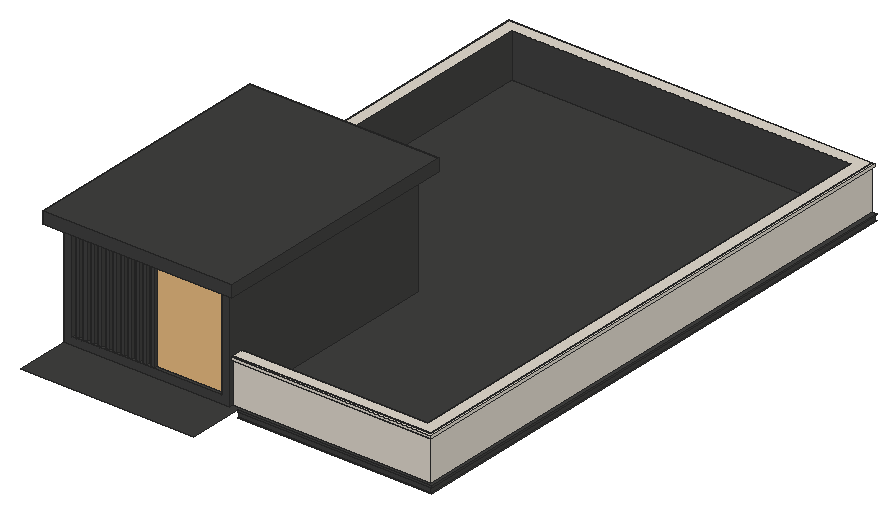
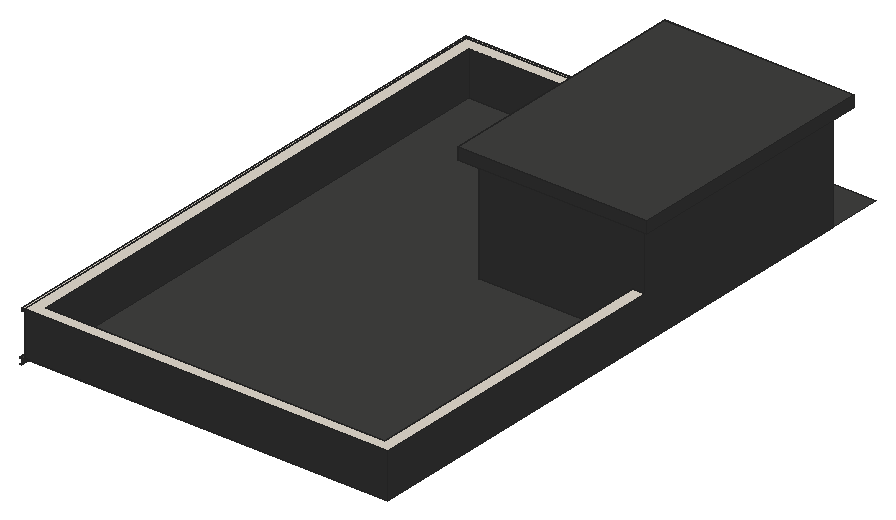
# SketchUp Ruby script. Lengths in inches.
U = 1.inch
M = Sketchup.active_model
def pt(a) = Geom::Point3d.new(a.map { |v| v * U })
def face(e, loops, mat)
  f = e.add_face(loops[0].map { |a| pt(a) })
  loops[1..].each { |l| e.add_face(l.map { |a| pt(a) }).erase! }
  f.material = f.back_material = mat if mat
  f
end
# faces: each face lists its corners as indices into pts; further lists are holes
def faces(e, pts, list, mat = nil) = list.each { |f| face(e, (f[0].is_a?(Array) ? f : [f]).map { |l| l.map { |i| pts[i] } }, mat) }
# xy, xz, yz: faces in a plane at the given z, y or x. An outline is a flat list of corners, or four numbers for a rectangle; further outlines are holes
def ring(l) = l.size == 4 ? [[l[0], l[1]], [l[2], l[1]], [l[2], l[3]], [l[0], l[3]]] : l.each_slice(2).to_a
def flat(e, list, mat, &to3) = list.each { |f| face(e, (f[0].is_a?(Array) ? f : [f]).map { |l| ring(l).map { |u, v| to3.(u, v) } }, mat) }
def xy(e, z, list, mat = nil) = flat(e, list, mat) { |x, y| [x, y, z] }
def xz(e, y, list, mat = nil) = flat(e, list, mat) { |x, z| [x, y, z] }
def yz(e, x, list, mat = nil) = flat(e, list, mat) { |y, z| [x, y, z] }
def lines(e, pts, list) = list.each { |a, b| e.add_line(pt(pts[a]), pt(pts[b])) }
# prism: a flat outline (further loops are holes) pulled along v
def prism(e, loops, v, mat = nil)
  f = face(e, loops, mat); d = Geom::Vector3d.new(v.map { |x| x * U })
  f.pushpull(f.normal.samedirection?(d) ? d.length : -d.length)
end
def box(e, o, s, mat = nil) = prism(e, [[o, [o[0] + s[0], o[1], o[2]], [o[0] + s[0], o[1] + s[1], o[2]], [o[0], o[1] + s[1], o[2]]]], [0, 0, s[2]], mat)
def at(x, y, z, deg = 0) = Geom::Transformation.translation(pt([x, y, z])) * Geom::Transformation.rotation(ORIGIN, Z_AXIS, deg.degrees)
def axes(o, x, y, z) = Geom::Transformation.new([*x, 0, *y, 0, *z, 0, *pt(o).to_a, 1])
def part(name) = M.definitions.add(name)
# library, detail: a bought-in or finely detailed component or shape, given as its bounding box
def library(name, o, s) = part(name).tap { |d| box(d.entities, o, s) }
def detail(e, o, s) = box(e.add_group.entities, o, s)
def put(e, d, t, mat = nil) = e.add_instance(d, t).tap { |i| i.material = mat if mat }
def group(e, t, mat = nil) = e.add_group.tap { |g| g.transformation = t; g.material = mat if mat }.entities
root = M.entities
M.materials.add("1448 AP 8253 RAVEN SONG").color = [64, 64, 63]
M.materials.add("Wall Light").color = [250, 218, 132]
M.materials.add("[Tile Various Tan]").color = [223, 216, 204]
c1 = part("2")
box(c1.entities,[0,0,0],[3,2,70])
c2 = library("PF4VTX2R\#1",[0,-0.39,0],[145.67,4.18,85.83])
xy(root,472,[[142.14,237,290.46,237,290.46,663,289.43,663,289.43,238,142.14,238]],"1448 AP 8253 RAVEN SONG")
xy(root,474,[[39.3,217.5,39.23,217.51,39.15,217.52,39.07,217.52,38.99,217.54,38.91,217.55,38.84,217.5625,38.76,217.58,38.68,217.6,38.61,217.62,38.53,217.64,38.39,217.7,38.3125,217.72,38.24,217.75,38.17,217.79,38.1,217.82,37.96,217.9,37.89,217.9375,37.83,217.98,37.76,218.02,37.7,218.07,37.63,218.11,37.45,218.26,37.23,218.48,37.18,218.54,37.125,218.6,37.08,218.66,37.03,218.73,36.98,218.79,36.94,218.86,36.9,218.92,36.78,219.13,36.75,219.2,36.71,219.27,36.65,219.41,36.625,219.49,36.6,219.5625,36.58,219.64,36.56,219.71,36.52,219.87,36.5,219.94,36.47,220.18,36.46,220.25,36.45,220.33,36.45,220.65,36.46,220.72,36.47,220.8,36.47,220.88,36.49,220.96,36.5,221.04,36.51,221.11,36.53,221.1875,36.55,221.27,36.57,221.34,36.59,221.42,36.62,221.49,36.65,221.5625,36.67,221.64,36.7,221.71,36.74,221.78,36.77,221.85,36.89,222.06,36.97,222.19,37.02,222.25,37.0625,222.32,37.11,222.38,37.21,222.5,37.32,222.61,37.375,222.67,37.43,222.72,37.55,222.82,37.61,222.875,37.68,222.92,37.74,222.97,37.81,223.01,37.87,223.05,38.08,223.17,38.15,223.2,38.22,223.24,38.36,223.3,38.4375,223.32,38.51,223.35,38.59,223.375,38.66,223.39,38.82,223.43,38.89,223.45,39.05,223.47,39.2,223.49,39.28,223.5,39.6,223.5,39.67,223.49,39.75,223.48,39.83,223.48,39.91,223.46,39.99,223.45,40.0625,223.4375,40.14,223.42,40.22,223.4,40.29,223.38,40.37,223.36,40.51,223.3,40.59,223.28,40.66,223.25,40.73,223.21,40.8,223.18,40.94,223.1,41.01,223.0625,41.07,223.02,41.14,222.98,41.2,222.93,41.27,222.89,41.45,222.74,41.51,222.68,41.5625,222.63,41.62,222.57,41.67,222.52,41.82,222.34,41.87,222.27,41.92,222.21,41.96,222.14,42,222.08,42.12,221.87,42.15,221.8,42.1875,221.73,42.22,221.66,42.25,221.59,42.27,221.51,42.3,221.4375,42.32,221.36,42.34,221.29,42.38,221.13,42.4,221.06,42.43,220.82,42.44,220.75,42.45,220.67,42.45,220.35,42.44,220.28,42.43,220.2,42.43,220.12,42.41,220.04,42.4,219.96,42.39,219.89,42.37,219.8125,42.35,219.73,42.33,219.66,42.31,219.58,42.28,219.51,42.25,219.4375,42.23,219.36,42.2,219.29,42.16,219.22,42.13,219.15,42.01,218.94,41.93,218.81,41.88,218.75,41.84,218.68,41.74,218.56,41.6875,218.5,41.63,218.44,41.47,218.28,41.35,218.18,41.29,218.125,41.22,218.08,41.16,218.03,41.09,217.99,41.03,217.95,40.82,217.83,40.75,217.8,40.68,217.76,40.54,217.7,40.46,217.68,40.39,217.65,40.3125,217.625,40.24,217.61,40.08,217.57,40.01,217.55,39.77,217.52,39.7,217.51,39.62,217.5],[117.99,217.5,117.92,217.51,117.84,217.52,117.76,217.52,117.68,217.54,117.6,217.55,117.53,217.5625,117.45,217.58,117.3,217.62,117.22,217.64,117.08,217.7,117,217.72,116.93,217.75,116.86,217.79,116.79,217.82,116.65,217.9,116.58,217.9375,116.52,217.98,116.45,218.02,116.39,218.07,116.32,218.11,116.14,218.26,115.92,218.48,115.77,218.66,115.72,218.73,115.67,218.79,115.63,218.86,115.59,218.92,115.47,219.13,115.4375,219.2,115.4,219.27,115.34,219.41,115.32,219.49,115.29,219.5625,115.27,219.64,115.25,219.71,115.21,219.87,115.19,219.94,115.16,220.18,115.15,220.25,115.14,220.33,115.14,220.65,115.15,220.72,115.16,220.8,115.16,220.88,115.18,220.96,115.1875,221.04,115.2,221.11,115.22,221.1875,115.24,221.27,115.26,221.34,115.28,221.42,115.31,221.49,115.34,221.5625,115.36,221.64,115.39,221.71,115.43,221.78,115.46,221.85,115.58,222.06,115.66,222.19,115.71,222.25,115.75,222.32,115.9,222.5,116.07,222.67,116.18,222.77,116.24,222.82,116.3,222.875,116.37,222.92,116.43,222.97,116.5,223.01,116.5625,223.05,116.63,223.09,116.77,223.17,116.84,223.2,116.91,223.24,117.05,223.3,117.13,223.32,117.2,223.35,117.28,223.375,117.35,223.39,117.51,223.43,117.58,223.45,117.82,223.48,117.89,223.49,117.97,223.5,118.29,223.5,118.36,223.49,118.44,223.48,118.52,223.48,118.6,223.46,118.68,223.45,118.75,223.4375,118.83,223.42,118.91,223.4,118.98,223.38,119.06,223.36,119.2,223.3,119.28,223.28,119.35,223.25,119.42,223.21,119.49,223.18,119.5625,223.14,119.63,223.1,119.7,223.0625,119.76,223.02,119.83,222.98,119.89,222.93,119.96,222.89,120.14,222.74,120.36,222.52,120.51,222.34,120.56,222.27,120.61,222.21,120.65,222.14,120.69,222.08,120.81,221.87,120.84,221.8,120.91,221.66,120.9375,221.59,120.96,221.51,120.99,221.4375,121.01,221.36,121.03,221.29,121.07,221.13,121.09,221.06,121.12,220.82,121.13,220.75,121.14,220.67,121.14,220.35,121.13,220.28,121.12,220.12,121.1,220.04,121.09,219.96,121.08,219.89,121.06,219.8125,121.04,219.73,121.02,219.66,121,219.58,120.97,219.51,120.94,219.4375,120.92,219.36,120.89,219.29,120.85,219.22,120.82,219.15,120.7,218.94,120.62,218.81,120.57,218.75,120.53,218.68,120.38,218.5,120.16,218.28,120.04,218.18,119.98,218.125,119.91,218.08,119.85,218.03,119.78,217.99,119.72,217.95,119.51,217.83,119.44,217.8,119.37,217.76,119.23,217.7,119.15,217.68,119.08,217.65,119,217.625,118.93,217.61,118.77,217.57,118.7,217.55,118.46,217.52,118.39,217.51,118.31,217.5]],"1448 AP 8253 RAVEN SONG")
xy(root,476,[[142.14,237,142.14,238,289.43,238,289.43,663,290.46,663,290.46,237]],"1448 AP 8253 RAVEN SONG")
xy(root,477,[[9.27,195,142.14,195,142.14,237,290.46,237,290.46,663,9.27,663]],"1448 AP 8253 RAVEN SONG")
xz(root,217.5,[[39.3,471,39.38,474],[39.38,471,39.46,474],[39.46,471,39.54,474],[39.54,471,39.62,474]],"1448 AP 8253 RAVEN SONG")
xz(root,217.52,[[39.07,471,39.15,474]],"1448 AP 8253 RAVEN SONG")
xz(root,223.48,[[39.75,471,39.83,474]],"1448 AP 8253 RAVEN SONG")
xz(root,223.5,[[39.28,471,39.36,474],[39.36,471,39.4375,474],[39.4375,471,39.52,474],[39.52,471,39.6,474]],"1448 AP 8253 RAVEN SONG")
xz(root,237,[[142.14,476,290.46,477]],"1448 AP 8253 RAVEN SONG")
xz(root,238,[[142.14,472,289.43,476]],"1448 AP 8253 RAVEN SONG")
yz(root,36.45,[[220.33,471,220.41,474],[220.41,471,220.49,474],[220.49,471,220.57,474],[220.57,471,220.65,474]],"1448 AP 8253 RAVEN SONG")
yz(root,36.47,[[220.8,471,220.88,474]],"1448 AP 8253 RAVEN SONG")
yz(root,42.43,[[220.12,471,220.2,474]],"1448 AP 8253 RAVEN SONG")
yz(root,42.45,[[220.35,471,220.43,474],[220.43,471,220.51,474],[220.51,471,220.59,474],[220.59,471,220.67,474]],"1448 AP 8253 RAVEN SONG")
yz(root,289.43,[[238,472,663,476]],"1448 AP 8253 RAVEN SONG")
yz(root,290.46,[[237,476,663,477]],"1448 AP 8253 RAVEN SONG")
p = [[38.91,217.55,471],[38.84,217.5625,471],[38.84,217.5625,474],[38.91,217.55,474],[38.99,217.54,471],[38.99,217.54,474],
  [39.07,217.52,471],[39.07,217.52,474],[39.23,217.51,471],[39.15,217.52,471],[39.15,217.52,474],[39.23,217.51,474],
  [39.3,217.5,471],[39.3,217.5,474],[39.7,217.51,471],[39.62,217.5,471],[39.62,217.5,474],[39.7,217.51,474],
  [39.77,217.52,471],[39.77,217.52,474],[39.85,217.53,471],[39.85,217.53,474],[40.01,217.55,471],[39.93,217.54,471],
  [39.93,217.54,474],[40.01,217.55,474],[38.61,217.62,471],[38.53,217.64,471],[38.53,217.64,474],[38.61,217.62,474],
  [38.46,217.67,471],[38.46,217.67,474],[38.68,217.6,471],[38.68,217.6,474],[38.76,217.58,471],[38.76,217.58,474],
  [40.08,217.57,471],[40.08,217.57,474],[40.16,217.59,471],[40.16,217.59,474],[40.3125,217.625,471],[40.24,217.61,471],
  [40.24,217.61,474],[40.3125,217.625,474],[40.39,217.65,471],[40.39,217.65,474],[38.3125,217.72,471],[38.24,217.75,471],
  [38.24,217.75,474],[38.3125,217.72,474],[38.39,217.7,471],[38.39,217.7,474],[40.46,217.68,471],[40.46,217.68,474],
  [40.61,217.73,471],[40.54,217.7,471],[40.54,217.7,474],[40.61,217.73,474],[40.68,217.76,471],[40.68,217.76,474],
  [38.1,217.82,471],[38.03,217.86,471],[38.03,217.86,474],[38.1,217.82,474],[38.17,217.79,471],[38.17,217.79,474],
  [40.75,217.8,471],[40.75,217.8,474],[40.89,217.87,471],[40.82,217.83,471],[40.82,217.83,474],[40.89,217.87,474],
  [37.89,217.9375,471],[37.83,217.98,471],[37.83,217.98,474],[37.89,217.9375,474],[37.96,217.9,471],[37.96,217.9,474],
  [40.96,217.91,471],[40.96,217.91,474],[41.09,217.99,471],[41.03,217.95,471],[41.03,217.95,474],[41.09,217.99,474],
  [37.76,218.02,471],[37.7,218.07,471],[37.7,218.07,474],[37.76,218.02,474],[41.16,218.03,471],[41.16,218.03,474],
  [41.22,218.08,471],[41.22,218.08,474],[37.63,218.11,471],[37.63,218.11,474],[37.57,218.16,471],[37.57,218.16,474],
  [41.29,218.125,471],[41.29,218.125,474],[41.35,218.18,471],[41.35,218.18,474],[37.51,218.21,471],[37.51,218.21,474],
  [37.45,218.26,471],[37.45,218.26,474],[41.41,218.23,471],[41.41,218.23,474],[41.47,218.28,471],[41.47,218.28,474],
  [37.39,218.32,471],[37.34,218.37,471],[37.34,218.37,474],[37.39,218.32,474],[41.58,218.39,471],[41.52,218.33,471],
  [41.52,218.33,474],[41.58,218.39,474],[37.28,218.43,471],[37.23,218.48,471],[37.23,218.48,474],[37.28,218.43,474],
  [41.6875,218.5,471],[41.63,218.44,471],[41.63,218.44,474],[41.6875,218.5,474],[37.18,218.54,471],[37.125,218.6,471],
  [37.125,218.6,474],[37.18,218.54,474],[41.74,218.56,471],[41.74,218.56,474],[37.08,218.66,471],[37.08,218.66,474],
  [41.79,218.62,471],[41.79,218.62,474],[41.84,218.68,471],[41.84,218.68,474],[37.03,218.73,471],[37.03,218.73,474],
  [36.98,218.79,471],[36.98,218.79,474],[41.88,218.75,471],[41.88,218.75,474],[41.93,218.81,471],[41.93,218.81,474],
  [36.94,218.86,471],[36.94,218.86,474],[41.97,218.875,471],[41.97,218.875,474],[36.9,218.92,471],[36.9,218.92,474],
  [36.86,218.99,471],[36.86,218.99,474],[42.05,219.01,471],[42.01,218.94,471],[42.01,218.94,474],[42.05,219.01,474],
  [36.82,219.06,471],[36.82,219.06,474],[42.09,219.08,471],[42.09,219.08,474],[36.78,219.13,471],[36.75,219.2,471],
  [36.75,219.2,474],[36.78,219.13,474],[42.16,219.22,471],[42.13,219.15,471],[42.13,219.15,474],[42.16,219.22,474],
  [36.71,219.27,471],[36.71,219.27,474],[42.2,219.29,471],[42.2,219.29,474],[36.68,219.34,471],[36.68,219.34,474],
  [36.65,219.41,471],[36.65,219.41,474],[42.23,219.36,471],[42.23,219.36,474],[36.625,219.49,471],[36.625,219.49,474],
  [42.25,219.4375,471],[42.25,219.4375,474],[42.28,219.51,471],[42.28,219.51,474],[36.6,219.5625,471],[36.6,219.5625,474],
  [42.31,219.58,471],[42.31,219.58,474],[36.58,219.64,471],[36.58,219.64,474],[36.56,219.71,471],[36.56,219.71,474],
  [42.33,219.66,471],[42.33,219.66,474],[36.54,219.79,471],[36.54,219.79,474],[42.35,219.73,471],[42.35,219.73,474],
  [42.37,219.8125,471],[42.37,219.8125,474],[36.52,219.87,471],[36.52,219.87,474],[42.39,219.89,471],[42.39,219.89,474],
  [36.5,219.94,471],[36.5,219.94,474],[36.49,220.02,471],[36.49,220.02,474],[42.4,219.96,471],[42.4,219.96,474],
  [36.48,220.1,471],[36.48,220.1,474],[42.43,220.12,471],[42.41,220.04,471],[42.41,220.04,474],[42.43,220.12,474],
  [36.47,220.18,471],[36.47,220.18,474],[36.46,220.25,471],[36.46,220.25,474],[42.44,220.28,471],[42.43,220.2,471],
  [42.43,220.2,474],[42.44,220.28,474],[36.45,220.33,471],[36.45,220.33,474],[42.45,220.35,471],[42.45,220.35,474],
  [36.45,220.65,471],[36.46,220.72,471],[36.46,220.72,474],[36.45,220.65,474],[36.47,220.8,471],[36.47,220.8,474],
  [42.43,220.82,471],[42.44,220.75,471],[42.44,220.75,474],[42.43,220.82,474],[42.45,220.67,471],[42.45,220.67,474],
  [42.42,220.9,471],[42.42,220.9,474],[36.47,220.88,471],[36.49,220.96,471],[36.49,220.96,474],[36.47,220.88,474],
  [42.41,220.98,471],[42.41,220.98,474],[36.5,221.04,471],[36.5,221.04,474],[36.51,221.11,471],[36.51,221.11,474],
  [42.4,221.06,471],[42.4,221.06,474],[36.53,221.1875,471],[36.53,221.1875,474],[42.36,221.21,471],[42.38,221.13,471],
  [42.38,221.13,474],[42.36,221.21,474],[36.55,221.27,471],[36.55,221.27,474],[42.34,221.29,471],[42.34,221.29,474],
  [36.57,221.34,471],[36.57,221.34,474],[36.59,221.42,471],[36.59,221.42,474],[42.32,221.36,471],[42.32,221.36,474],
  [36.62,221.49,471],[36.62,221.49,474],[42.27,221.51,471],[42.3,221.4375,471],[42.3,221.4375,474],[42.27,221.51,474],
  [36.65,221.5625,471],[36.65,221.5625,474],[42.25,221.59,471],[42.25,221.59,474],[36.67,221.64,471],[36.67,221.64,474],
  [36.7,221.71,471],[36.7,221.71,474],[42.22,221.66,471],[42.22,221.66,474],[36.74,221.78,471],[36.74,221.78,474],
  [42.15,221.8,471],[42.1875,221.73,471],[42.1875,221.73,474],[42.15,221.8,474],[36.77,221.85,471],[36.77,221.85,474],
  [42.12,221.87,471],[42.12,221.87,474],[36.81,221.92,471],[36.81,221.92,474],[36.85,221.99,471],[36.85,221.99,474],
  [42.04,222.01,471],[42.08,221.94,471],[42.08,221.94,474],[42.04,222.01,474],[36.89,222.06,471],[36.89,222.06,474],
  [42,222.08,471],[42,222.08,474],[36.93,222.125,471],[36.93,222.125,474],[36.97,222.19,471],[36.97,222.19,474],
  [41.92,222.21,471],[41.96,222.14,471],[41.96,222.14,474],[41.92,222.21,474],[37.02,222.25,471],[37.02,222.25,474],
  [41.87,222.27,471],[41.87,222.27,474],[37.0625,222.32,471],[37.0625,222.32,474],[37.11,222.38,471],[37.11,222.38,474],
  [41.77,222.4,471],[41.82,222.34,471],[41.82,222.34,474],[41.77,222.4,474],[37.16,222.44,471],[37.16,222.44,474],
  [37.21,222.5,471],[37.21,222.5,474],[41.72,222.46,471],[41.72,222.46,474],[37.27,222.56,471],[37.27,222.56,474],
  [41.62,222.57,471],[41.67,222.52,471],[41.67,222.52,474],[41.62,222.57,474],[37.32,222.61,471],[37.32,222.61,474],
  [37.375,222.67,471],[37.375,222.67,474],[41.51,222.68,471],[41.5625,222.63,471],[41.5625,222.63,474],[41.51,222.68,474],
  [37.43,222.72,471],[37.43,222.72,474],[37.49,222.77,471],[37.49,222.77,474],[41.39,222.79,471],[41.45,222.74,471],
  [41.45,222.74,474],[41.39,222.79,474],[37.55,222.82,471],[37.55,222.82,474],[37.61,222.875,471],[37.61,222.875,474],
  [41.27,222.89,471],[41.33,222.84,471],[41.33,222.84,474],[41.27,222.89,474],[37.68,222.92,471],[37.68,222.92,474],
  [37.74,222.97,471],[37.74,222.97,474],[41.14,222.98,471],[41.2,222.93,471],[41.2,222.93,474],[41.14,222.98,474],
  [37.81,223.01,471],[37.81,223.01,474],[37.87,223.05,471],[37.87,223.05,474],[41.01,223.0625,471],[41.07,223.02,471],
  [41.07,223.02,474],[41.01,223.0625,474],[37.94,223.09,471],[37.94,223.09,474],[38.01,223.13,471],[38.01,223.13,474],
  [38.08,223.17,471],[38.08,223.17,474],[40.8,223.18,471],[40.87,223.14,471],[40.87,223.14,474],[40.8,223.18,474],
  [40.94,223.1,471],[40.94,223.1,474],[38.15,223.2,471],[38.15,223.2,474],[38.22,223.24,471],[38.22,223.24,474],
  [38.29,223.27,471],[38.29,223.27,474],[40.59,223.28,471],[40.66,223.25,471],[40.66,223.25,474],[40.59,223.28,474],
  [40.73,223.21,471],[40.73,223.21,474],[119.28,223.28,471],[119.35,223.25,471],[119.35,223.25,474],[119.28,223.28,474],
  [119.42,223.21,471],[119.42,223.21,474],[119.49,223.18,471],[119.49,223.18,474],[38.36,223.3,471],[38.36,223.3,474],
  [38.4375,223.32,471],[38.4375,223.32,474],[38.51,223.35,471],[38.51,223.35,474],[38.59,223.375,471],[38.59,223.375,474],
  [40.37,223.36,471],[40.44,223.33,471],[40.44,223.33,474],[40.37,223.36,474],[40.51,223.3,471],[40.51,223.3,474],
  [119.06,223.36,471],[119.13,223.33,471],[119.13,223.33,474],[119.06,223.36,474],[119.2,223.3,471],[119.2,223.3,474],
  [38.66,223.39,471],[38.66,223.39,474],[38.74,223.41,471],[38.74,223.41,474],[38.82,223.43,471],[38.82,223.43,474],
  [38.89,223.45,471],[38.89,223.45,474],[38.97,223.46,471],[38.97,223.46,474],[39.99,223.45,471],[40.0625,223.4375,471],
  [40.0625,223.4375,474],[39.99,223.45,474],[40.14,223.42,471],[40.14,223.42,474],[40.22,223.4,471],[40.22,223.4,474],
  [40.29,223.38,471],[40.29,223.38,474],[118.83,223.42,471],[118.91,223.4,471],[118.91,223.4,474],[118.83,223.42,474],
  [118.98,223.38,471],[118.98,223.38,474],[39.05,223.47,471],[39.05,223.47,474],[39.125,223.48,471],[39.125,223.48,474],
  [39.2,223.49,471],[39.2,223.49,474],[39.28,223.5,471],[39.28,223.5,474],[39.6,223.5,471],[39.67,223.49,471],
  [39.67,223.49,474],[39.6,223.5,474],[39.75,223.48,471],[39.75,223.48,474],[39.83,223.48,471],[39.91,223.46,471],
  [39.91,223.46,474],[39.83,223.48,474]]
faces(root,p,[[0,1,2,3],[4,0,3,5],[6,4,5,7],[8,9,10,11],[12,8,11,13],[14,15,16,17],[18,14,17,19],[20,18,19,21],
  [22,23,24,25],[23,20,21,24],[26,27,28,29],[27,30,31,28],[32,26,29,33],[34,32,33,35],[1,34,35,2],[36,22,25,37],
  [38,36,37,39],[40,41,42,43],[41,38,39,42],[44,40,43,45],[46,47,48,49],[50,46,49,51],[30,50,51,31],[52,44,45,53],
  [54,55,56,57],[55,52,53,56],[58,54,57,59],[60,61,62,63],[64,60,63,65],[47,64,65,48],[66,58,59,67],[68,69,70,71],
  [69,66,67,70],[72,73,74,75],[76,72,75,77],[61,76,77,62],[78,68,71,79],[80,81,82,83],[81,78,79,82],[84,85,86,87],
  [73,84,87,74],[88,80,83,89],[90,88,89,91],[85,92,93,86],[92,94,95,93],[96,90,91,97],[98,96,97,99],[94,100,101,95],
  [100,102,103,101],[104,98,99,105],[106,104,105,107],[108,109,110,111],[102,108,111,103],[112,113,114,115],[113,106,107,114],[116,117,118,119],
  [109,116,119,110],[120,121,122,123],[121,112,115,122],[124,125,126,127],[117,124,127,118],[128,120,123,129],[125,130,131,126],[132,128,129,133],
  [134,132,133,135],[130,136,137,131],[136,138,139,137],[140,134,135,141],[142,140,141,143],[138,144,145,139],[146,142,143,147],[144,148,149,145],
  [148,150,151,149],[152,153,154,155],[153,146,147,154],[150,156,157,151],[158,152,155,159],[160,161,162,163],[156,160,163,157],[164,165,166,167],
  [165,158,159,166],[161,168,169,162],[170,164,167,171],[168,172,173,169],[172,174,175,173],[176,170,171,177],[174,178,179,175],[180,176,177,181],
  [182,180,181,183],[178,184,185,179],[186,182,183,187],[184,188,189,185],[188,190,191,189],[192,186,187,193],[190,194,195,191],[196,192,193,197],
  [198,196,197,199],[194,200,201,195],[202,198,199,203],[200,204,205,201],[204,206,207,205],[208,202,203,209],[206,210,211,207],[212,213,214,215],
  [213,208,209,214],[210,216,217,211],[216,218,219,217],[220,221,222,223],[218,224,225,219],[226,220,223,227],[228,229,230,231],[229,232,233,230],
  [234,235,236,237],[235,238,239,236],[240,234,237,241],[242,243,244,245],[246,240,241,247],[243,248,249,244],[248,250,251,249],[252,246,247,253],
  [250,254,255,251],[256,257,258,259],[257,252,253,258],[254,260,261,255],[262,256,259,263],[260,264,265,261],[264,266,267,265],[268,262,263,269],
  [266,270,271,267],[272,273,274,275],[273,268,269,274],[270,276,277,271],[278,272,275,279],[276,280,281,277],[280,282,283,281],[284,278,279,285],
  [282,286,287,283],[288,289,290,291],[289,284,285,290],[286,292,293,287],[294,288,291,295],[292,296,297,293],[296,298,299,297],[300,301,302,303],
  [301,294,295,302],[298,304,305,299],[306,300,303,307],[304,308,309,305],[308,310,311,309],[312,313,314,315],[313,306,307,314],[310,316,317,311],
  [318,312,315,319],[316,320,321,317],[320,322,323,321],[324,325,326,327],[325,318,319,326],[322,328,329,323],[328,330,331,329],[332,324,327,333],
  [330,334,335,331],[336,337,338,339],[337,332,333,338],[334,340,341,335],[340,342,343,341],[344,345,346,347],[345,336,339,346],[342,348,349,343],
  [348,350,351,349],[352,353,354,355],[353,344,347,354],[350,356,357,351],[356,358,359,357],[360,361,362,363],[361,352,355,362],[358,364,365,359],
  [364,366,367,365],[368,369,370,371],[369,360,363,370],[366,372,373,367],[372,374,375,373],[376,377,378,379],[377,368,371,378],[374,380,381,375],
  [380,382,383,381],[382,384,385,383],[386,387,388,389],[387,390,391,388],[390,376,379,391],[384,392,393,385],[392,394,395,393],[394,396,397,395],
  [398,399,400,401],[399,402,403,400],[402,386,389,403],[404,405,406,407],[405,408,409,406],[408,410,411,409],[396,412,413,397],[412,414,415,413],
  [414,416,417,415],[416,418,419,417],[420,421,422,423],[421,424,425,422],[424,398,401,425],[426,427,428,429],[427,430,431,428],[430,404,407,431],
  [418,432,433,419],[432,434,435,433],[434,436,437,435],[436,438,439,437],[438,440,441,439],[442,443,444,445],[443,446,447,444],[446,448,449,447],
  [448,450,451,449],[450,420,423,451],[452,453,454,455],[453,456,457,454],[456,426,429,457],[440,458,459,441],[458,460,461,459],[460,462,463,461],
  [462,464,465,463],[466,467,468,469],[467,470,471,468],[472,473,474,475],[473,442,445,474]],"1448 AP 8253 RAVEN SONG")
g1 = group(root,at(9.27,240,477),"1448 AP 8253 RAVEN SONG")
xy(g1,0,[[[0,-3,0,423,278.1,423,278.1,0,126.69,0,126.69,-3],[126.69,9,268.83,9,268.83,414,9.27,414,9.27,177,126.69,177],[6.18,6,120.51,171]]])
xy(g1,6,[[6.18,-3,120.51,6]])
xy(g1,30.875,[[126.81,0,277.98,0.25]],"[Tile Various Tan]")
xy(g1,31.875,[[126.81,0,277.98,0.25]],"[Tile Various Tan]")
xy(g1,32,[[126.69,-2,126.69,0,278.1,0,278.1,423,280.16,423,280.16,-2]],"[Tile Various Tan]")
xy(g1,34,[[126.69,-2,280.16,-2,280.16,423,278.1,423,278.1,0,126.69,0],[126.69,0,278.1,0,278.1,423,0,423,0,177,9.27,177,9.27,414,268.83,414,268.83,9,126.69,9]],"[Tile Various Tan]")
xy(g1,76,[[6.18,-3,120.51,6]])
xy(g1,82,[[[0,-3,126.69,177],[6.18,6,120.51,171]]])
xz(g1,-3,[[[0,0,126.69,82],[6.18,6,120.51,76]]])
xz(g1,-2,[[126.69,32,280.16,34]],"[Tile Various Tan]")
xz(g1,0,[[126.69,32,278.1,34]])
xz(g1,0,[[[126.69,0,278.1,32],[126.81,30.875,277.98,31.875]]],"[Tile Various Tan]")
xz(g1,0.25,[[126.81,30.875,277.98,31.875]],"[Tile Various Tan]")
xz(g1,6,[[6.18,0,120.51,6],[6.18,76,120.51,82]])
xz(g1,9,[[126.69,0,268.83,34]])
xz(g1,171,[[6.18,0,120.51,82]])
xz(g1,177,[[9.27,0,9.27,34,0,34,0,82,126.69,82,126.69,0]])
xz(g1,414,[[9.27,0,268.83,34]])
xz(g1,423,[[0,0,278.1,34],[278.1,32,280.16,34]])
yz(g1,0,[[-3,0,-3,82,177,82,177,34,423,34,423,0]])
yz(g1,6.18,[[6,0,171,0,171,82,6,82,6,76,-3,76,-3,6,6,6]])
yz(g1,9.27,[[177,0,414,34]])
yz(g1,120.51,[[6,0,171,82],[-3,6,6,76]])
yz(g1,126.69,[[-3,0,0,0,0,32,-2,32,-2,34,9,34,9,0,177,0,177,82,-3,82],[-2,32,0,34]])
yz(g1,126.81,[[0,30.875,0.25,31.875]],"[Tile Various Tan]")
yz(g1,268.83,[[9,0,414,34]])
yz(g1,277.98,[[0,30.875,0.25,31.875]],"[Tile Various Tan]")
yz(g1,278.1,[[0,32,423,34]])
yz(g1,278.1,[[0,0,423,32]],"[Tile Various Tan]")
yz(g1,280.16,[[-2,32,423,34]],"[Tile Various Tan]")
put(g1,c1,axes([7.72,-1.5,6],[1.03,0,0],[0,1,0],[0,0,1]))
put(g1,c1,axes([13.45,-1.5,6],[1.03,0,0],[0,1,0],[0,0,1]))
put(g1,c1,axes([19.17,-1.5,6],[1.03,0,0],[0,1,0],[0,0,1]))
put(g1,c1,axes([24.89,-1.5,6],[1.03,0,0],[0,1,0],[0,0,1]))
put(g1,c1,axes([30.62,-1.5,6],[1.03,0,0],[0,1,0],[0,0,1]))
put(g1,c1,axes([36.34,-1.5,6],[1.03,0,0],[0,1,0],[0,0,1]))
put(g1,c1,axes([42.0625,-1.5,6],[1.03,0,0],[0,1,0],[0,0,1]))
put(g1,c1,axes([47.79,-1.5,6],[1.03,0,0],[0,1,0],[0,0,1]))
put(g1,c1,axes([53.51,-1.5,6],[1.03,0,0],[0,1,0],[0,0,1]))
put(g1,c1,axes([59.23,-1.5,6],[1.03,0,0],[0,1,0],[0,0,1]))
put(g1,c1,axes([64.95,-1.5,6],[1.03,0,0],[0,1,0],[0,0,1]))
g2 = group(g1,at(0,-3,82))
box(g2,[-9.27,-9,0],[145.23,198,9])
g3 = group(g1,at(126.81,0,30.875),"Wall Light")
box(g3,[0,0,0],[151.16,0.25,1],"Wall Light")
put(root,c2,axes([15.45,241,483],[0.78486,0,0],[0,1,0],[0,0,0.8156]))
